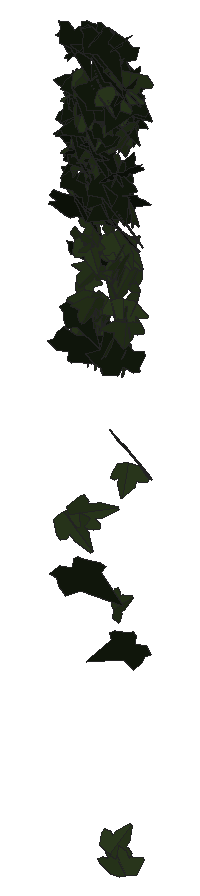
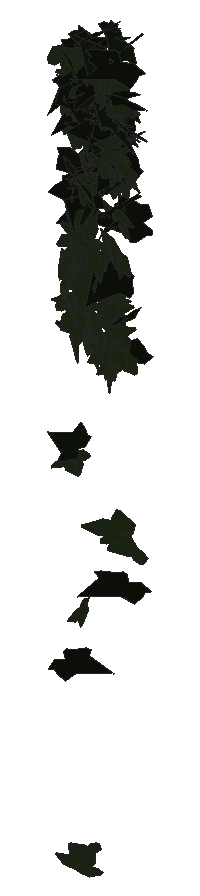
# SketchUp Ruby script. Lengths in inches.
U = 1.inch
M = Sketchup.active_model
def pt(a) = Geom::Point3d.new(a.map { |v| v * U })
def face(e, loops, mat)
  f = e.add_face(loops[0].map { |a| pt(a) })
  loops[1..].each { |l| e.add_face(l.map { |a| pt(a) }).erase! }
  f.material = f.back_material = mat if mat
  f
end
# faces: each face lists its corners as indices into pts; further lists are holes
def faces(e, pts, list, mat = nil) = list.each { |f| face(e, (f[0].is_a?(Array) ? f : [f]).map { |l| l.map { |i| pts[i] } }, mat) }
# xy, xz, yz: faces in a plane at the given z, y or x. An outline is a flat list of corners, or four numbers for a rectangle; further outlines are holes
def ring(l) = l.size == 4 ? [[l[0], l[1]], [l[2], l[1]], [l[2], l[3]], [l[0], l[3]]] : l.each_slice(2).to_a
def flat(e, list, mat, &to3) = list.each { |f| face(e, (f[0].is_a?(Array) ? f : [f]).map { |l| ring(l).map { |u, v| to3.(u, v) } }, mat) }
def xy(e, z, list, mat = nil) = flat(e, list, mat) { |x, y| [x, y, z] }
def xz(e, y, list, mat = nil) = flat(e, list, mat) { |x, z| [x, y, z] }
def yz(e, x, list, mat = nil) = flat(e, list, mat) { |y, z| [x, y, z] }
def lines(e, pts, list) = list.each { |a, b| e.add_line(pt(pts[a]), pt(pts[b])) }
# prism: a flat outline (further loops are holes) pulled along v
def prism(e, loops, v, mat = nil)
  f = face(e, loops, mat); d = Geom::Vector3d.new(v.map { |x| x * U })
  f.pushpull(f.normal.samedirection?(d) ? d.length : -d.length)
end
def box(e, o, s, mat = nil) = prism(e, [[o, [o[0] + s[0], o[1], o[2]], [o[0] + s[0], o[1] + s[1], o[2]], [o[0], o[1] + s[1], o[2]]]], [0, 0, s[2]], mat)
def at(x, y, z, deg = 0) = Geom::Transformation.translation(pt([x, y, z])) * Geom::Transformation.rotation(ORIGIN, Z_AXIS, deg.degrees)
def axes(o, x, y, z) = Geom::Transformation.new([*x, 0, *y, 0, *z, 0, *pt(o).to_a, 1])
def part(name) = M.definitions.add(name)
# library, detail: a bought-in or finely detailed component or shape, given as its bounding box
def library(name, o, s) = part(name).tap { |d| box(d.entities, o, s) }
def detail(e, o, s) = box(e.add_group.entities, o, s)
def put(e, d, t, mat = nil) = e.add_instance(d, t).tap { |i| i.material = mat if mat }
def group(e, t, mat = nil) = e.add_group.tap { |g| g.transformation = t; g.material = mat if mat }.entities
root = M.entities
M.materials.add("1026 AP 7946 SUNNY SIDE UP").color = [254, 231, 186]
M.materials.add("efeu1").color = [18, 25, 13]
M.materials.add("efeu2").color = [43, 57, 29]
c1 = part("ivyleaf_9")
p = [[1.54,2.16,1.25],[1.36,2.04,1.19],[-0.21,0.99,0.68],[-0.71,1.11,0.82],[-0.85,0.86,0.67],[-0.8,0.17,0.21],
  [-0.9,-0.01,0.1],[-0.67,-0.16,-0.02],[-0.08,-0.08,-0.05],[-0.03,-0.6,-0.4],[0.65,-0.88,-0.66],[0.83,-0.6,-0.49],
  [1.29,-0.42,-0.43],[1.8125,-0.07,-0.26],[1.21,0.44,0.15]]
faces(c1.entities,p,[[0,1,2,3,4,5,6,7,8,9,10,11,12,13,14]],"efeu1")
c2 = part("ivyleaf_10")
p = [[0,0.5,-0.03],[-0.0625,2.02,-0.43],[-0.19,2.01,-0.46],[-0.54,1.05,-0.29],[-0.52,0.625,-0.18],[-0.83,0.76,-0.28],
  [-1.16,0.64,-0.33],[-1.15,0.33,-0.24],[-0.77,-0.39,0.02],[-0.3,-0.51,0.16],[0.04,-0.48,0.23],[-0.02,2.01,-0.4375],
  [-0.06,2.01,-0.43],[0.04,-0.49,0.23],[0.67,-0.49,0.14],[1.38,0.36,-0.2],[1.375,0.51,-0.24],[0.81,0.65,-0.19],
  [0.62,0.59,-0.15],[0.6,1.09,-0.28],[0.5,1.23,-0.31]]
faces(c2.entities,p,[[0,1,2,3,4,5,6,7,8,9,10],[11,12,0,13,14,15,16,17,18,19,20]],"efeu2")
put(root,c1,axes([110.64,212.89,264.78],[0.02301,-0.24408,-0.02449],[-0.00562,0.02221,-0.25176],[0.38536,0.0149,-0.00221]),"1026 AP 7946 SUNNY SIDE UP")
put(root,c2,axes([110.81,212.84,265.49],[-0.16708,-0.22222,0],[0.01007,-0.00446,-0.25366],[0.34928,-0.10617,0.00731]),"1026 AP 7946 SUNNY SIDE UP")
put(root,c2,axes([110.79,212.82,263.62],[-0.33314,0.10245,-0.00138],[-0.01182,-0.01994,-0.24157],[-0.16069,-0.21094,0.02063]),"1026 AP 7946 SUNNY SIDE UP")
put(root,c2,axes([110.78,212.88,265.5625],[0.36444,-0.08859,-0.02862],[-0.05525,-0.01598,-0.25416],[0.13488,0.23283,-0.02677]),"1026 AP 7946 SUNNY SIDE UP")
put(root,c2,axes([110.68,212.9,266],[0.14164,0.21599,0.09352],[0.0499,0.08379,-0.24058],[-0.36425,0.09546,0.00341]),"1026 AP 7946 SUNNY SIDE UP")
put(root,c2,axes([110.83,212.81,265.36],[-0.01238,-0.24169,0.06161],[-0.00736,-0.06105,-0.24946],[0.39195,-0.00878,-0.00274]),"1026 AP 7946 SUNNY SIDE UP")
put(root,c1,axes([110.71,212.86,265.97],[-0.06946,-0.24263,0.05661],[0.00018,-0.05722,-0.25418],[0.39165,-0.043,0.01016]),"1026 AP 7946 SUNNY SIDE UP")
put(root,c1,axes([110.48,212.5625,264.35],[0.31118,-0.00843,0.16356],[0.24632,-0.03344,-0.20312],[0.04317,0.25153,-0.02002]),"1026 AP 7946 SUNNY SIDE UP")
put(root,c2,axes([110.69,212.83,261.7],[-0.21562,-0.1084,-0.14852],[0.20161,0.0677,-0.17845],[0.19838,-0.18662,0.01993]),"1026 AP 7946 SUNNY SIDE UP")
put(root,c1,axes([110.97,212.91,266.57],[-0.18792,0.21618,-0.05031],[0.02264,-0.04919,-0.25451],[-0.34818,-0.11987,0.01061]),"1026 AP 7946 SUNNY SIDE UP")
put(root,c2,axes([110.78,212.86,261.59],[-0.17289,0.18791,-0.05492],[0.00074,-0.06213,-0.22251],[-0.3076,-0.10577,0.03033]),"1026 AP 7946 SUNNY SIDE UP")
put(root,c1,axes([110.89,212.83,265.52],[-0.29917,0.08822,-0.13447],[0.15953,-0.08897,-0.214],[-0.19037,-0.2132,0.03198]),"1026 AP 7946 SUNNY SIDE UP")
put(root,c2,axes([110.77,212.88,262.76],[0.0529,0.22478,-0.03497],[-0.00733,-0.03492,-0.23435],[-0.35769,0.03396,-0.00037]),"1026 AP 7946 SUNNY SIDE UP")
put(root,c2,axes([110.85,212.83,266.47],[-0.17026,-0.21656,0.07777],[0.0292,-0.09278,-0.24336],[0.36007,-0.09487,0.05651]),"1026 AP 7946 SUNNY SIDE UP")
put(root,c2,axes([110.85,212.82,262.06],[-0.10808,-0.17949,0.13618],[0.03017,-0.14359,-0.18996],[0.35017,-0.04303,0.0584]),"1026 AP 7946 SUNNY SIDE UP")
put(root,c2,axes([110.54,212.71,257.92],[0.24999,0.0168,0.22162],[0.33912,-0.01551,-0.16312],[0.00397,0.26697,-0.02185]),"1026 AP 7946 SUNNY SIDE UP")
put(root,c2,axes([110.81,212.81,265.89],[0.2721,-0.17823,0.05052],[0.02871,-0.05175,-0.25517],[0.28967,0.17255,-0.02216]),"1026 AP 7946 SUNNY SIDE UP")
put(root,c2,axes([110.86,212.82,264.53],[0.33084,-0.11235,-0.03225],[-0.05449,0.00006,-0.24516],[0.17483,0.21263,-0.01538]),"1026 AP 7946 SUNNY SIDE UP")
put(root,c1,axes([110.67,212.86,266.34],[0.12575,-0.23815,0.04023],[0.00124,-0.0423,-0.25873],[0.37982,0.07898,-0.01248]),"1026 AP 7946 SUNNY SIDE UP")
put(root,c1,axes([110.94,212.88,266.41],[-0.37992,0.00571,-0.07421],[0.11192,-0.02525,-0.24804],[-0.01991,-0.25087,0.02179]),"1026 AP 7946 SUNNY SIDE UP")
put(root,c2,axes([110.83,212.85,265.39],[0.2607,-0.18745,-0.01035],[0.02477,0.02585,-0.25593],[0.29405,0.16401,0.03074]),"1026 AP 7946 SUNNY SIDE UP")
put(root,c2,axes([110.8,212.99,261.9375],[0.00201,0.21825,-0.05239],[-0.00139,-0.05209,-0.22514],[-0.35281,0.00145,0.00059]),"1026 AP 7946 SUNNY SIDE UP")
put(root,c2,axes([110.78,212.87,265.58],[0.18104,0.20476,0.08844],[0.04434,0.08112,-0.24108],[-0.34559,0.11767,0.0154]),"1026 AP 7946 SUNNY SIDE UP")
put(root,c2,axes([110.87,212.64,266.33],[-0.01261,0.24784,0.017],[-0.03599,0.0143,-0.25433],[-0.38876,-0.00936,0.023]),"1026 AP 7946 SUNNY SIDE UP")
put(root,c1,axes([110.72,212.68,267.78],[0.08156,-0.26174,0.01228],[-0.00055,-0.01373,-0.27495],[0.4121,0.05178,-0.0028]),"1026 AP 7946 SUNNY SIDE UP")
put(root,c1,axes([110.65,212.97,267.64],[-0.03474,-0.06747,-0.27753],[0.21699,0.23142,-0.07012],[0.37829,-0.13894,0.01473]),"1026 AP 7946 SUNNY SIDE UP")
put(root,c1,axes([110.62,212.83,265.35],[0.02658,-0.08173,0.24303],[0.25803,-0.17517,-0.07551],[0.29679,0.15961,0.04388]),"1026 AP 7946 SUNNY SIDE UP")
put(root,c1,axes([110.98,212.78,266.73],[-0.3798,-0.09129,-0.03064],[0.05414,-0.00869,-0.26525],[0.14067,-0.24315,0.01936]),"1026 AP 7946 SUNNY SIDE UP")
put(root,c2,axes([111.12,212.57,265.35],[0.14657,-0.04315,-0.23838],[-0.29022,0.14063,-0.1029],[0.22909,0.20577,0.02216]),"1026 AP 7946 SUNNY SIDE UP")
put(root,c2,axes([110.92,212.93,261.54],[0.20611,-0.16518,-0.08548],[-0.00714,0.09773,-0.20961],[0.28992,0.11984,0.05561]),"1026 AP 7946 SUNNY SIDE UP")
put(root,c1,axes([110.78,212.86,263.375],[0.41369,0.03882,-0.04426],[-0.06124,-0.03069,-0.273],[-0.06773,0.26484,-0.02354]),"1026 AP 7946 SUNNY SIDE UP")
put(root,c2,axes([111.01,212.88,263.07],[-0.14051,-0.16793,0.1347],[-0.06145,-0.12749,-0.19553],[0.3299,-0.09527,0.02095]),"1026 AP 7946 SUNNY SIDE UP")
put(root,c1,axes([110.89,212.61,265.54],[0.19185,0.22423,0.08485],[0.08104,0.06413,-0.26221],[-0.36606,0.13171,-0.01358]),"1026 AP 7946 SUNNY SIDE UP")
put(root,c2,axes([110.97,212.77,262.52],[-0.12913,-0.20636,0.09137],[0.00599,-0.09692,-0.22626],[0.35386,-0.07367,0.03717]),"1026 AP 7946 SUNNY SIDE UP")
put(root,c1,axes([110.8125,212.58,262.34],[0.10805,-0.20078,-0.12464],[-0.0504,0.11565,-0.21786],[0.36421,0.07557,0.00683]),"1026 AP 7946 SUNNY SIDE UP")
put(root,c1,axes([110.84,212.65,264.49],[0.25301,-0.15494,-0.10326],[-0.13464,0.05379,-0.22898],[0.25619,0.18129,-0.01837]),"1026 AP 7946 SUNNY SIDE UP")
put(root,c2,axes([110.8,212.95,261.82],[-0.26621,-0.05119,-0.14537],[0.23416,-0.03408,-0.17189],[0.02596,-0.21756,0.05976]),"1026 AP 7946 SUNNY SIDE UP")
put(root,c1,axes([110.73,212.86,265.27],[0.24742,-0.19302,-0.01498],[0.0206,0.02792,-0.25479],[0.30354,0.15544,0.02951]),"1026 AP 7946 SUNNY SIDE UP")
put(root,c2,axes([110.95,212.92,261.56],[-0.20954,0.169,-0.07147],[-0.00596,-0.08953,-0.21474],[-0.28777,-0.12121,0.05649]),"1026 AP 7946 SUNNY SIDE UP")
put(root,c2,axes([110.98,212.87,262.24],[0.28737,-0.13049,-0.02403],[-0.03736,0.00556,-0.23112],[0.20486,0.18407,-0.00843]),"1026 AP 7946 SUNNY SIDE UP")
put(root,c1,axes([110.74,212.51,261.48],[-0.04864,0.02007,0.24921],[0.38146,-0.00115,0.03207],[0.00581,0.24376,-0.01893]),"1026 AP 7946 SUNNY SIDE UP")
put(root,c2,axes([111.01,212.77,265.29],[-0.09431,-0.23668,0.01086],[0.01003,-0.01387,-0.25142],[0.37248,-0.05955,0.00952]),"1026 AP 7946 SUNNY SIDE UP")
put(root,c2,axes([110.8,212.7,258.14],[-0.06894,-0.05354,0.26794],[0.17636,0.23554,0.07073],[-0.37898,0.11935,-0.01582]),"1026 AP 7946 SUNNY SIDE UP")
put(root,c2,axes([111,212.82,263.93],[0.27399,-0.15814,-0.05467],[-0.04101,0.04866,-0.24141],[0.25861,0.17526,0.01963]),"1026 AP 7946 SUNNY SIDE UP")
put(root,c1,axes([111.04,212.38,267.67],[0.10742,0.16537,0.20102],[0.00581,0.20037,-0.17595],[-0.40102,0.0472,0.0513]),"1026 AP 7946 SUNNY SIDE UP")
put(root,c2,axes([110.97,212.99,262.07],[-0.04857,0.21157,-0.07176],[-0.02675,-0.07356,-0.21906],[-0.34982,-0.02375,0.02672]),"1026 AP 7946 SUNNY SIDE UP")
put(root,c1,axes([110.6875,212.81,266.14],[0.23551,-0.00687,0.20644],[0.31487,0.01871,-0.15339],[-0.01714,0.24951,0.01865]),"1026 AP 7946 SUNNY SIDE UP")
put(root,c1,axes([111.18,212.83,266.23],[-0.38069,-0.0562,0.05767],[-0.06792,-0.05857,-0.25195],[0.10503,-0.24157,0.0461]),"1026 AP 7946 SUNNY SIDE UP")
put(root,c1,axes([111.16,212.9,266.34],[-0.39283,0.00186,-0.0135],[0.01913,-0.06605,-0.24866],[-0.00826,-0.2413,0.06645]),"1026 AP 7946 SUNNY SIDE UP")
put(root,c1,axes([110.82,212.8125,265.37],[0.06942,-0.24085,-0.01952],[0.05896,0.02449,-0.24852],[0.37512,0.04072,0.04268]),"1026 AP 7946 SUNNY SIDE UP")
put(root,c1,axes([110.875,212.84,266.33],[0.01808,-0.25082,0.04363],[0.00444,-0.04369,-0.25892],[0.40032,0.01181,0.0009]),"1026 AP 7946 SUNNY SIDE UP")
put(root,c2,axes([111.09,212.83,267.03],[-0.16617,0.19934,0.11371],[-0.11692,0.08353,-0.23063],[-0.33776,-0.12698,0.02389]),"1026 AP 7946 SUNNY SIDE UP")
put(root,c1,axes([110.8,212.57,257.08],[0.02332,-0.09747,-0.25773],[0.17908,0.2286,-0.08365],[0.38142,-0.10137,0.05503]),"1026 AP 7946 SUNNY SIDE UP")
put(root,c2,axes([111,212.6,267.01],[-0.02433,-0.20536,-0.16254],[0.12114,0.14608,-0.20432],[0.38761,-0.05855,0.05365]),"1026 AP 7946 SUNNY SIDE UP")
put(root,c2,axes([111.14,212.67,266.39],[-0.36077,0.08312,0.04877],[-0.09592,-0.0339,-0.24589],[-0.11539,-0.23171,0.05191]),"1026 AP 7946 SUNNY SIDE UP")
put(root,c2,axes([110.98,212.66,267.03],[0.18157,0.21496,0.07688],[0.01776,0.07681,-0.24958],[-0.35673,0.11323,0.02671]),"1026 AP 7946 SUNNY SIDE UP")
put(root,c1,axes([111,212.8,266.78],[-0.15823,-0.23057,-0.02182],[0.02553,0.01459,-0.25892],[0.363,-0.10153,0.00869]),"1026 AP 7946 SUNNY SIDE UP")
put(root,c2,axes([111.04,212.92,262.4],[-0.06716,0.22214,0.00542],[-0.00696,0.00322,-0.23299],[-0.34928,-0.04278,0.0036]),"1026 AP 7946 SUNNY SIDE UP")
put(root,c1,axes([110.89,212.88,265.68],[0.10945,-0.24015,0.01701],[0.01806,-0.01527,-0.25758],[0.37822,0.07022,0.00738]),"1026 AP 7946 SUNNY SIDE UP")
put(root,c2,axes([111.11,212.93,263.54],[-0.14394,-0.21541,0.03411],[0.00955,-0.03973,-0.24038],[0.34285,-0.08933,0.02101]),"1026 AP 7946 SUNNY SIDE UP")
put(root,c2,axes([111.1,212.75,265.44],[0.20509,-0.20761,-0.01031],[-0.02897,-0.00117,-0.25204],[0.32545,0.13072,-0.01594]),"1026 AP 7946 SUNNY SIDE UP")
put(root,c2,axes([111.13,212.65,262.53],[-0.11157,-0.21288,0.0743],[-0.00925,-0.07511,-0.23092],[0.35391,-0.06907,0.01739]),"1026 AP 7946 SUNNY SIDE UP")
put(root,c2,axes([111.11,212.85,266.95],[0.0091,-0.25863,-0.02122],[0.0145,0.01933,-0.26621],[0.40753,0.00509,0.00994]),"1026 AP 7946 SUNNY SIDE UP")
put(root,c1,axes([110.98,212.64,266.23],[0.34265,0.11715,-0.00953],[0.00171,-0.02289,-0.25412],[-0.18485,0.21693,-0.02001]),"1026 AP 7946 SUNNY SIDE UP")
put(root,c2,axes([110.91,212.77,263.58],[0.2871,-0.02354,0.15742],[0.23148,-0.04645,-0.1887],[0.07496,0.23361,-0.02022]),"1026 AP 7946 SUNNY SIDE UP")
put(root,c1,axes([111.45,212.72,266.25],[-0.40999,0.00839,0.0913],[-0.13989,-0.02284,-0.26772],[-0.00089,-0.27443,0.02346]),"1026 AP 7946 SUNNY SIDE UP")
put(root,c2,axes([111.24,212.96,262.25],[0.02265,-0.2263,0.01932],[-0.01059,-0.0205,-0.23358],[0.35708,0.01375,-0.00815]),"1026 AP 7946 SUNNY SIDE UP")
put(root,c1,axes([111.14,212.81,266.06],[0.04839,0.07406,0.2484],[0.24433,0.18525,-0.0781],[-0.31163,0.15674,-0.02266]),"1026 AP 7946 SUNNY SIDE UP")
put(root,c2,axes([111.17,212.625,266.22],[0.17069,0.22717,-0.02862],[-0.00359,-0.03109,-0.2593],[-0.3601,0.10799,-0.01098]),"1026 AP 7946 SUNNY SIDE UP")
put(root,c2,axes([111.3,212.64,266.34],[-0.30136,0.16446,0.02967],[-0.06414,-0.00505,-0.25834],[-0.25433,-0.19361,0.03]),"1026 AP 7946 SUNNY SIDE UP")
put(root,c2,axes([111.2,212.93,265.1],[0.1695,0.20083,0.09365],[0.00785,0.0977,-0.2308],[-0.3458,0.10066,0.04067]),"1026 AP 7946 SUNNY SIDE UP")
put(root,c1,axes([111.21,212.63,266.44],[0.34618,0.09349,-0.06799],[-0.07945,-0.05026,-0.2453],[-0.162,0.22444,-0.025]),"1026 AP 7946 SUNNY SIDE UP")
put(root,c2,axes([111.3,212.99,262.36],[0.12071,-0.21321,-0.01386],[0.00441,0.01402,-0.23324],[0.33577,0.07646,0.00805]),"1026 AP 7946 SUNNY SIDE UP")
put(root,c1,axes([111.11,212.82,267.86],[0.15761,-0.23096,-0.08463],[0.00007,0.08737,-0.2566],[0.38476,0.09459,0.03471]),"1026 AP 7946 SUNNY SIDE UP")
put(root,c1,axes([111.4,212.72,267.63],[0.09008,0.20438,0.14372],[-0.03372,0.14561,-0.21161],[-0.38661,0.03492,0.05194]),"1026 AP 7946 SUNNY SIDE UP")
put(root,c1,axes([111.21,212.9,265.01],[-0.11445,-0.23117,-0.0159],[0.07657,-0.00081,-0.24502],[0.35604,-0.07414,0.04759]),"1026 AP 7946 SUNNY SIDE UP")
put(root,c1,axes([111.16,212.8,265.68],[0.1688,-0.22151,-0.02344],[-0.0145,0.01941,-0.25347],[0.34964,0.10775,0.0008]),"1026 AP 7946 SUNNY SIDE UP")
put(root,c2,axes([111.37,212.92,261.89],[0.0601,-0.22265,0.03293],[-0.00124,-0.03384,-0.23283],[0.35397,0.03768,-0.00641]),"1026 AP 7946 SUNNY SIDE UP")
put(root,c1,axes([111.1875,212.95,266.84],[0.24792,-0.1837,-0.07146],[-0.0711,0.05123,-0.2491],[0.29987,0.16402,0.00002]),"1026 AP 7946 SUNNY SIDE UP")
put(root,c1,axes([111.45,212.63,266.71],[-0.31752,-0.12499,0.12939],[0.16188,0.07355,0.24496],[-0.22774,0.22654,-0.00627]),"1026 AP 7946 SUNNY SIDE UP")
put(root,c1,axes([111.55,212.96,265.1],[-0.0685,0.19139,0.15078],[-0.09126,0.13489,-0.20021],[-0.36663,-0.06933,0.02166]),"1026 AP 7946 SUNNY SIDE UP")
put(root,c2,axes([111.375,212.82,265.1875],[0.17735,-0.21599,0.01711],[-0.00142,-0.02058,-0.25092],[0.34078,0.11232,-0.00995]),"1026 AP 7946 SUNNY SIDE UP")
put(root,c2,axes([111.42,212.9,264.28],[-0.09685,-0.23384,0.00528],[0.01158,-0.00861,-0.24898],[0.36764,-0.06133,0.00923]),"1026 AP 7946 SUNNY SIDE UP")
put(root,c1,axes([111.15,212.88,266.53],[0.21553,-0.18104,0.11321],[0.07507,-0.10236,-0.2335],[0.3253,0.14357,-0.02112]),"1026 AP 7946 SUNNY SIDE UP")
put(root,c2,axes([111.35,212.87,262.79],[-0.10407,0.21258,-0.05755],[0.0149,-0.05678,-0.22956],[-0.34577,-0.06643,0.00743]),"1026 AP 7946 SUNNY SIDE UP")
put(root,c2,axes([111.44,212.85,265.92],[-0.08465,-0.24713,-0.01113],[0.00027,0.00958,-0.2605],[0.38888,-0.0538,-0.00224]),"1026 AP 7946 SUNNY SIDE UP")
put(root,c1,axes([111.45,212.87,265],[-0.23849,-0.17199,0.09348],[-0.05412,-0.09076,-0.23449],[0.30167,-0.15225,0.03183]),"1026 AP 7946 SUNNY SIDE UP")
put(root,c2,axes([111.5,212.96,262.99],[-0.34403,-0.05358,0.03722],[-0.04914,-0.02512,-0.23156],[0.08924,-0.22038,0.01596]),"1026 AP 7946 SUNNY SIDE UP")
put(root,c1,axes([111.35,212.93,265.25],[-0.08185,-0.2402,0.00905],[0.00678,-0.01132,-0.25317],[0.37797,-0.05181,0.0065]),"1026 AP 7946 SUNNY SIDE UP")
put(root,c1,axes([111.57,213.23,255.56],[-0.02132,-0.02901,-0.25084],[-0.03545,-0.24251,0.02966],[-0.38368,0.02402,0.0112]),"1026 AP 7946 SUNNY SIDE UP")
put(root,c1,axes([111.52,212.91,266.14],[-0.36416,-0.09378,-0.02576],[0.05144,-0.01595,-0.256],[0.14345,-0.23234,0.02639]),"1026 AP 7946 SUNNY SIDE UP")
put(root,c2,axes([111.52,212.8125,266.66],[-0.21006,-0.19498,0.08963],[-0.03114,-0.09216,-0.24157],[0.33499,-0.13083,0.03375]),"1026 AP 7946 SUNNY SIDE UP")
put(root,c1,axes([111.6875,212.82,267.5],[-0.11605,-0.00139,0.25126],[-0.35877,-0.08968,-0.07218],[0.13556,-0.23853,0.02408]),"1026 AP 7946 SUNNY SIDE UP")
put(root,c1,axes([111.28,212.7,267.9],[0.06659,-0.25971,-0.06541],[0.01257,0.064,-0.27009],[0.41966,0.03929,0.01847]),"1026 AP 7946 SUNNY SIDE UP")
put(root,c2,axes([111.52,212.92,263.43],[-0.35279,-0.06123,0.02038],[-0.02116,-0.0268,-0.23865],[0.09911,-0.22366,0.02159]),"1026 AP 7946 SUNNY SIDE UP")
put(root,c1,axes([111.4,212.87,265.01],[-0.09584,-0.23886,0.01697],[0.00273,-0.01883,-0.25399],[0.37662,-0.06065,0.00616]),"1026 AP 7946 SUNNY SIDE UP")
put(root,c2,axes([111.52,212.86,265.3125],[0.14306,-0.21446,-0.09071],[-0.02075,0.08835,-0.23851],[0.36323,0.08952,0.0221]),"1026 AP 7946 SUNNY SIDE UP")
put(root,c2,axes([111.59,212.97,263.41],[-0.22337,-0.14538,0.11785],[-0.05031,-0.12376,-0.20221],[0.28732,-0.13469,0.05622]),"1026 AP 7946 SUNNY SIDE UP")
put(root,c1,axes([111.57,212.84,264.62],[-0.23994,-0.13796,0.13286],[-0.0787,-0.13132,-0.20527],[0.28721,-0.15125,0.05474]),"1026 AP 7946 SUNNY SIDE UP")
put(root,c2,axes([111.55,212.89,266.41],[-0.2091,-0.18755,0.10253],[0.00704,-0.12106,-0.22712],[0.33456,-0.11467,0.06886]),"1026 AP 7946 SUNNY SIDE UP")
put(root,c2,axes([111.42,212.87,251.58],[0.15184,0.12574,-0.18574],[0.12938,0.16277,0.16265],[0.3215,-0.12489,0.02227]),"1026 AP 7946 SUNNY SIDE UP")
put(root,c2,axes([111.49,212.86,256.46],[0.0413,-0.02728,-0.23702],[0.07188,0.22745,-0.02109],[0.35689,-0.04265,0.03168]),"1026 AP 7946 SUNNY SIDE UP")
put(root,c1,axes([111.32,212.65,267.41],[0.26426,-0.19586,-0.04124],[-0.0432,0.02771,-0.2657],[0.31101,0.17027,-0.00186]),"1026 AP 7946 SUNNY SIDE UP")
put(root,c1,axes([111.62,212.84,266.64],[0.03053,0.25077,-0.0553],[-0.0042,-0.05506,-0.25944],[-0.4037,0.01954,-0.00148]),"1026 AP 7946 SUNNY SIDE UP")
put(root,c2,axes([111.57,212.7,261.62],[0.22891,-0.17483,-0.04978],[-0.06637,0.0263,-0.23369],[0.27696,0.1508,-0.01486]),"1026 AP 7946 SUNNY SIDE UP")
put(root,c1,axes([111.48,212.81,266.98],[0.35349,-0.00211,-0.12078],[-0.18427,0.0041,-0.23156],[0.00593,0.2535,0.00423]),"1026 AP 7946 SUNNY SIDE UP")
put(root,c2,axes([111.59,212.85,267.41],[-0.01451,-0.25975,0.01503],[0.00024,-0.01608,-0.26785],[0.40921,-0.0092,0.00069]),"1026 AP 7946 SUNNY SIDE UP")
put(root,c2,axes([111.58,212.6,261.93],[0.09771,-0.22382,-0.06437],[-0.00704,0.0622,-0.23862],[0.3648,0.06115,0.01264]),"1026 AP 7946 SUNNY SIDE UP")
put(root,c2,axes([111.63,212.85,251.26],[0.32094,0.09309,0.09296],[-0.14368,-0.01471,0.22982],[0.14379,-0.22246,0.02217]),"1026 AP 7946 SUNNY SIDE UP")
put(root,c2,axes([111.58,212.78,266.38],[-0.11083,-0.21909,0.11195],[0.04204,-0.12056,-0.2306],[0.38312,-0.05015,0.05769]),"1026 AP 7946 SUNNY SIDE UP")
put(root,c2,axes([111.58,212.9,263.42],[0.05237,-0.1321,0.24449],[-0.09307,0.2306,0.14169],[-0.41787,-0.06791,-0.00091]),"1026 AP 7946 SUNNY SIDE UP")
put(root,c2,axes([111.57,212.9,266.07],[0.34032,-0.12626,-0.00673],[-0.02685,-0.01778,-0.25705],[0.19692,0.21578,-0.02342]),"1026 AP 7946 SUNNY SIDE UP")
put(root,c2,axes([111.61,212.89,263.43],[0.01868,-0.22704,0.05019],[0.00705,-0.04984,-0.2345],[0.36549,0.01256,0.00196]),"1026 AP 7946 SUNNY SIDE UP")
put(root,c1,axes([111.51,212.8,266.45],[0.02762,-0.04518,-0.25894],[-0.09932,0.24309,-0.04819],[0.38868,0.06533,0.00609]),"1026 AP 7946 SUNNY SIDE UP")
put(root,c1,axes([111.6,212.78,264.68],[0.2128,0.1997,-0.04161],[-0.01585,-0.04323,-0.24825],[-0.32034,0.1348,-0.01536]),"1026 AP 7946 SUNNY SIDE UP")
put(root,c2,axes([111.625,212.93,263.28],[0.02655,-0.15781,-0.17822],[0.02802,0.17292,-0.16054],[0.36609,-0.00179,0.02521]),"1026 AP 7946 SUNNY SIDE UP")
put(root,c1,axes([111.72,212.76,265.29],[0.01539,0.23743,-0.05814],[-0.01636,-0.05738,-0.24501],[-0.38389,0.01197,0.00811]),"1026 AP 7946 SUNNY SIDE UP")
put(root,c1,axes([111.51,212.71,265.07],[-0.06399,-0.21869,-0.11013],[0.02677,0.1043,-0.22854],[0.38097,-0.04406,-0.00244]),"1026 AP 7946 SUNNY SIDE UP")
put(root,c2,axes([111.67,212.91,262.18],[-0.17201,-0.19956,0.01326],[0.0046,-0.01756,-0.23428],[0.31453,-0.10888,0.01068]),"1026 AP 7946 SUNNY SIDE UP")
put(root,c1,axes([111.44,212.87,264.48],[0.29643,-0.15295,-0.01689],[-0.0425,-0.0088,-0.24893],[0.23796,0.18895,-0.02343]),"1026 AP 7946 SUNNY SIDE UP")
put(root,c1,axes([111.46,212.76,266.63],[0.05823,-0.22494,-0.12033],[0.05077,0.12001,-0.22936],[0.39437,0.01777,0.0473]),"1026 AP 7946 SUNNY SIDE UP")
put(root,c1,axes([111.86,212.69,267.07],[-0.26214,0.09389,-0.20573],[-0.25693,0.11668,0.1972],[0.23433,0.23296,-0.01393]),"1026 AP 7946 SUNNY SIDE UP")
put(root,c2,axes([111.72,212.91,263.21],[-0.19325,-0.18115,0.08058],[-0.01481,-0.08784,-0.22242],[0.31056,-0.11692,0.03954]),"1026 AP 7946 SUNNY SIDE UP")
put(root,c2,axes([111.74,212.9,266.51],[-0.00789,-0.25127,-0.01103],[-0.00309,0.00932,-0.25884],[0.39535,-0.00494,-0.00224]),"1026 AP 7946 SUNNY SIDE UP")
put(root,c2,axes([111.625,212.88,262.52],[0.30829,0.1171,0.01372],[0.02505,-0.00203,-0.23506],[-0.1835,0.19646,-0.00904]),"1026 AP 7946 SUNNY SIDE UP")
put(root,c2,axes([111.49,212.84,263.83],[0.28555,0.01533,0.16371],[0.25088,-0.01477,-0.18656],[-0.00278,0.2408,-0.02044]),"1026 AP 7946 SUNNY SIDE UP")
put(root,c1,axes([111.74,212.82,266.84],[-0.32252,-0.15271,-0.03878],[0.07732,-0.00498,-0.26126],[0.23457,-0.20833,0.0328]),"1026 AP 7946 SUNNY SIDE UP")
put(root,c2,axes([111.81,212.75,262.4],[-0.15559,0.18843,0.08936],[-0.13112,0.05062,-0.21362],[-0.29789,-0.1207,0.04736]),"1026 AP 7946 SUNNY SIDE UP")
put(root,c2,axes([111.75,213.05,262.61],[0.18218,-0.19598,0.01164],[-0.00476,-0.01619,-0.23437],[0.30874,0.1154,-0.01048]),"1026 AP 7946 SUNNY SIDE UP")
put(root,c1,axes([111.91,212.5,261.61],[-0.398,-0.03085,0.02911],[0.03956,0.02756,0.26167],[-0.0528,0.25321,-0.02342]),"1026 AP 7946 SUNNY SIDE UP")
put(root,c2,axes([111.49,212.86,263.76],[0.2176,0.06578,0.19289],[0.29118,0.03802,-0.15485],[-0.11066,0.2294,-0.02816]),"1026 AP 7946 SUNNY SIDE UP")
put(root,c2,axes([111.78,212.78,263.61],[0.08724,-0.22859,0.01507],[0.00198,-0.01608,-0.24241],[0.3603,0.05544,-0.00232]),"1026 AP 7946 SUNNY SIDE UP")
put(root,c2,axes([111.64,212.65,266.88],[0.33048,0.12461,0.06029],[0.08352,0.02374,-0.25149],[-0.1992,0.21668,-0.00542]),"1026 AP 7946 SUNNY SIDE UP")
put(root,c2,axes([111.83,212.85,264.63],[-0.22086,0.1869,0.07641],[-0.10969,0.03821,-0.23847],[-0.2959,-0.15367,0.03136]),"1026 AP 7946 SUNNY SIDE UP")
put(root,c2,axes([111.73,212.87,261.67],[0.1303,-0.20153,0.06726],[0.07625,-0.05144,-0.2234],[0.32483,0.09292,0.02546]),"1026 AP 7946 SUNNY SIDE UP")
put(root,c1,axes([111.53,212.76,264.2],[0.11224,-0.14539,0.18566],[0.14183,-0.15717,-0.16759],[0.33643,0.11476,0.00871]),"1026 AP 7946 SUNNY SIDE UP")
put(root,c2,axes([111.8,212.99,263.31],[0.19354,-0.194,-0.00772],[-0.01805,0.00028,-0.23649],[0.30469,0.12325,-0.0091]),"1026 AP 7946 SUNNY SIDE UP")
put(root,c2,axes([111.84,212.83,266.05],[-0.00884,-0.25247,-0.03792],[-0.0014,0.0354,-0.25994],[0.40086,-0.00544,-0.00174]),"1026 AP 7946 SUNNY SIDE UP")
put(root,c1,axes([111.76,212.77,266.83],[0.05446,-0.0951,-0.24398],[-0.14023,0.21884,-0.10292],[0.37515,0.09561,-0.00306]),"1026 AP 7946 SUNNY SIDE UP")
put(root,c2,axes([111.85,212.78,266.68],[0.16979,-0.23059,-0.03446],[-0.02293,0.02866,-0.26213],[0.36536,0.10895,-0.00043]),"1026 AP 7946 SUNNY SIDE UP")
put(root,c2,axes([111.79,212.8125,259.3125],[0.18054,0.18873,-0.07083],[-0.04973,-0.06247,-0.22789],[-0.31249,0.11898,-0.00466]),"1026 AP 7946 SUNNY SIDE UP")
put(root,c1,axes([111.57,212.98,259.66],[0.14445,-0.17365,0.15376],[0.13405,-0.12446,-0.20262],[0.33525,0.12459,0.01477]),"1026 AP 7946 SUNNY SIDE UP")
put(root,c2,axes([111.92,212.74,267.28],[-0.32715,-0.14538,0.02637],[-0.01777,-0.02985,-0.261],[0.23166,-0.20759,0.01722]),"1026 AP 7946 SUNNY SIDE UP")
put(root,c2,axes([111.89,212.8,266.25],[0.02108,-0.23776,0.07931],[-0.00038,-0.07846,-0.24574],[0.39362,0.01266,-0.00449]),"1026 AP 7946 SUNNY SIDE UP")
put(root,c2,axes([111.91,212.62,262.33],[-0.24402,-0.169,0.00971],[0.00605,-0.0176,-0.23599],[0.26617,-0.15454,0.01426]),"1026 AP 7946 SUNNY SIDE UP")
